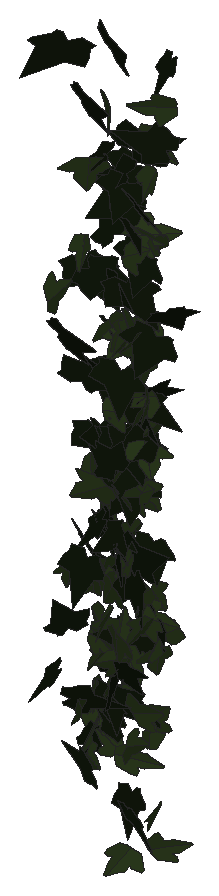
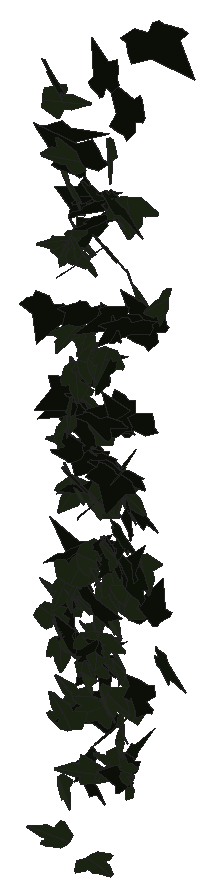
# SketchUp Ruby script. Lengths in inches.
U = 1.inch
M = Sketchup.active_model
def pt(a) = Geom::Point3d.new(a.map { |v| v * U })
def face(e, loops, mat)
  f = e.add_face(loops[0].map { |a| pt(a) })
  loops[1..].each { |l| e.add_face(l.map { |a| pt(a) }).erase! }
  f.material = f.back_material = mat if mat
  f
end
# faces: each face lists its corners as indices into pts; further lists are holes
def faces(e, pts, list, mat = nil) = list.each { |f| face(e, (f[0].is_a?(Array) ? f : [f]).map { |l| l.map { |i| pts[i] } }, mat) }
# xy, xz, yz: faces in a plane at the given z, y or x. An outline is a flat list of corners, or four numbers for a rectangle; further outlines are holes
def ring(l) = l.size == 4 ? [[l[0], l[1]], [l[2], l[1]], [l[2], l[3]], [l[0], l[3]]] : l.each_slice(2).to_a
def flat(e, list, mat, &to3) = list.each { |f| face(e, (f[0].is_a?(Array) ? f : [f]).map { |l| ring(l).map { |u, v| to3.(u, v) } }, mat) }
def xy(e, z, list, mat = nil) = flat(e, list, mat) { |x, y| [x, y, z] }
def xz(e, y, list, mat = nil) = flat(e, list, mat) { |x, z| [x, y, z] }
def yz(e, x, list, mat = nil) = flat(e, list, mat) { |y, z| [x, y, z] }
def lines(e, pts, list) = list.each { |a, b| e.add_line(pt(pts[a]), pt(pts[b])) }
# prism: a flat outline (further loops are holes) pulled along v
def prism(e, loops, v, mat = nil)
  f = face(e, loops, mat); d = Geom::Vector3d.new(v.map { |x| x * U })
  f.pushpull(f.normal.samedirection?(d) ? d.length : -d.length)
end
def box(e, o, s, mat = nil) = prism(e, [[o, [o[0] + s[0], o[1], o[2]], [o[0] + s[0], o[1] + s[1], o[2]], [o[0], o[1] + s[1], o[2]]]], [0, 0, s[2]], mat)
def at(x, y, z, deg = 0) = Geom::Transformation.translation(pt([x, y, z])) * Geom::Transformation.rotation(ORIGIN, Z_AXIS, deg.degrees)
def axes(o, x, y, z) = Geom::Transformation.new([*x, 0, *y, 0, *z, 0, *pt(o).to_a, 1])
def part(name) = M.definitions.add(name)
# library, detail: a bought-in or finely detailed component or shape, given as its bounding box
def library(name, o, s) = part(name).tap { |d| box(d.entities, o, s) }
def detail(e, o, s) = box(e.add_group.entities, o, s)
def put(e, d, t, mat = nil) = e.add_instance(d, t).tap { |i| i.material = mat if mat }
def group(e, t, mat = nil) = e.add_group.tap { |g| g.transformation = t; g.material = mat if mat }.entities
root = M.entities
M.materials.add("1026 AP 7946 SUNNY SIDE UP").color = [254, 231, 186]
M.materials.add("efeu1").color = [18, 25, 13]
M.materials.add("efeu2").color = [43, 57, 29]
c1 = part("ivyleaf_9")
p = [[1.54,2.16,1.25],[1.36,2.04,1.19],[-0.21,0.99,0.68],[-0.71,1.11,0.82],[-0.85,0.86,0.67],[-0.8,0.17,0.21],
  [-0.9,-0.01,0.1],[-0.67,-0.16,-0.02],[-0.08,-0.08,-0.05],[-0.03,-0.6,-0.4],[0.65,-0.88,-0.66],[0.83,-0.6,-0.49],
  [1.29,-0.42,-0.43],[1.8125,-0.07,-0.26],[1.21,0.44,0.15]]
faces(c1.entities,p,[[0,1,2,3,4,5,6,7,8,9,10,11,12,13,14]],"efeu1")
c2 = part("ivyleaf_10")
p = [[0,0.5,-0.03],[-0.0625,2.02,-0.43],[-0.19,2.01,-0.46],[-0.54,1.05,-0.29],[-0.52,0.625,-0.18],[-0.83,0.76,-0.28],
  [-1.16,0.64,-0.33],[-1.15,0.33,-0.24],[-0.77,-0.39,0.02],[-0.3,-0.51,0.16],[0.04,-0.48,0.23],[-0.02,2.01,-0.4375],
  [-0.06,2.01,-0.43],[0.04,-0.49,0.23],[0.67,-0.49,0.14],[1.38,0.36,-0.2],[1.375,0.51,-0.24],[0.81,0.65,-0.19],
  [0.62,0.59,-0.15],[0.6,1.09,-0.28],[0.5,1.23,-0.31]]
faces(c2.entities,p,[[0,1,2,3,4,5,6,7,8,9,10],[11,12,0,13,14,15,16,17,18,19,20]],"efeu2")
put(root,c1,axes([112.84,209.66,257.05],[-0.37781,-0.01782,-0.19523],[0.29911,-0.02649,-0.24619],[-0.00391,-0.3048,0.031]),"1026 AP 7946 SUNNY SIDE UP")
put(root,c1,axes([112.12,209.95,267.53],[0.03774,0.15785,-0.31881],[-0.06989,-0.30717,-0.16628],[-0.54303,0.0505,-0.00076]),"1026 AP 7946 SUNNY SIDE UP")
put(root,c1,axes([111.9375,210.06,261.28],[0.36942,-0.04727,-0.20032],[0.3095,0.00278,0.24465],[-0.05447,-0.30479,0.03148]),"1026 AP 7946 SUNNY SIDE UP")
put(root,c1,axes([111.83,210.03,254.21],[-0.27818,0.12757,-0.14576],[0.15899,-0.10192,-0.22437],[-0.25487,-0.20282,0.01912]),"1026 AP 7946 SUNNY SIDE UP")
put(root,c1,axes([112.01,210.17,255.13],[0.1892,0.0973,0.21691],[-0.29272,-0.09995,0.15701],[0.21625,-0.22043,0.02275]),"1026 AP 7946 SUNNY SIDE UP")
put(root,c1,axes([113.27,210.39,251.58],[0.18124,-0.20702,0.06487],[0.03095,-0.06236,-0.24411],[0.33938,0.11624,-0.01239]),"1026 AP 7946 SUNNY SIDE UP")
put(root,c2,axes([111.68,210.08,261.99],[0.03216,0.01268,-0.31587],[0.09557,0.30111,0.01876],[0.47309,-0.06169,0.01768]),"1026 AP 7946 SUNNY SIDE UP")
put(root,c2,axes([111.97,210.4,256.37],[-0.05548,-0.27655,0.01769],[0.00326,-0.01915,-0.28729],[0.43584,-0.03506,0.0044]),"1026 AP 7946 SUNNY SIDE UP")
put(root,c1,axes([112.28,210.46,252.09],[0.07837,-0.24976,0.04331],[0.0022,0.04456,0.26244],[-0.39862,-0.04886,0.00996]),"1026 AP 7946 SUNNY SIDE UP")
put(root,c2,axes([112.04,210.59,253.21],[-0.05761,-0.19311,-0.1727],[-0.02026,-0.16664,0.201],[-0.40046,0.03621,0.01467]),"1026 AP 7946 SUNNY SIDE UP")
put(root,c1,axes([112.03,210.59,266],[0.34896,-0.09762,-0.19804],[0.31181,-0.01386,0.24372],[-0.13105,-0.29292,0.05255]),"1026 AP 7946 SUNNY SIDE UP")
put(root,c2,axes([112.98,210.43,255.11],[-0.33435,0.15157,0.06874],[-0.10884,0.01577,-0.26753],[-0.23596,-0.22205,0.026]),"1026 AP 7946 SUNNY SIDE UP")
put(root,c1,axes([112.84,210.66,260.55],[-0.12699,-0.28062,-0.00455],[0.019,-0.00055,-0.30059],[0.44087,-0.08081,0.01165]),"1026 AP 7946 SUNNY SIDE UP")
put(root,c1,axes([111.92,210.43,253.47],[0.22646,0.03739,0.22439],[0.3424,0.01889,-0.15171],[-0.05738,0.26026,-0.01967]),"1026 AP 7946 SUNNY SIDE UP")
put(root,c2,axes([113.29,210.37,253],[-0.02217,-0.10445,-0.24966],[0.10453,0.23284,-0.10627],[0.40067,-0.06652,0.01391]),"1026 AP 7946 SUNNY SIDE UP")
put(root,c1,axes([112.625,210.7,253.7],[0.04338,0.11867,0.27502],[-0.12079,-0.25506,0.12381],[0.4422,-0.08131,0.00684]),"1026 AP 7946 SUNNY SIDE UP")
put(root,c2,axes([112.4,210.63,257.99],[-0.26989,-0.0335,0.21812],[-0.3125,-0.07742,-0.17889],[0.1271,-0.26149,0.02333]),"1026 AP 7946 SUNNY SIDE UP")
put(root,c2,axes([113.35,210.74,255.42],[-0.00839,-0.21307,0.16183],[-0.00922,-0.1582,-0.22049],[0.41727,-0.00778,-0.00162]),"1026 AP 7946 SUNNY SIDE UP")
put(root,c2,axes([112.68,210.85,254.4],[-0.00264,0.07244,0.29267],[0.05489,-0.28161,0.07265],[0.45709,0.03424,-0.00703]),"1026 AP 7946 SUNNY SIDE UP")
put(root,c2,axes([112.46,210.76,255.29],[0.14967,-0.25162,0.0702],[0.02316,-0.06876,-0.27734],[0.40983,0.09578,-0.00997]),"1026 AP 7946 SUNNY SIDE UP")
put(root,c2,axes([112.97,210.76,263],[0.1487,-0.16465,-0.18246],[0.22404,-0.11452,0.18838],[-0.30591,-0.16391,0.04927]),"1026 AP 7946 SUNNY SIDE UP")
put(root,c2,axes([113.52,210.57,260.18],[0.12239,-0.21871,-0.18692],[-0.03173,0.18212,-0.23563],[0.44446,0.07323,0.03465]),"1026 AP 7946 SUNNY SIDE UP")
put(root,c1,axes([112.28,210.79,257.17],[-0.29222,0.11367,-0.13312],[0.1565,-0.08531,-0.22417],[-0.2217,-0.21006,0.01721]),"1026 AP 7946 SUNNY SIDE UP")
put(root,c1,axes([112.95,210.84,251.65],[-0.27007,-0.00097,-0.21958],[0.33276,-0.03334,-0.17573],[-0.03987,-0.27169,0.02073]),"1026 AP 7946 SUNNY SIDE UP")
put(root,c1,axes([112.73,210.61,258.52],[-0.06344,0.11746,0.2405],[-0.21429,0.19132,-0.12267],[-0.34953,-0.13861,0.03155]),"1026 AP 7946 SUNNY SIDE UP")
put(root,c1,axes([112.97,210.89,264.03],[0.18064,-0.158,0.17429],[0.14243,-0.14422,-0.20189],[0.33609,0.14603,-0.00812]),"1026 AP 7946 SUNNY SIDE UP")
put(root,c1,axes([112.67,210.71,254.3],[0.37853,0.07605,-0.02641],[-0.02774,-0.03032,-0.25913],[-0.12333,0.24023,-0.02278]),"1026 AP 7946 SUNNY SIDE UP")
put(root,c2,axes([112.98,211.01,261.03],[-0.0252,-0.02202,-0.27195],[-0.0797,-0.2592,0.02394],[-0.40863,0.05191,0.0121]),"1026 AP 7946 SUNNY SIDE UP")
put(root,c1,axes([112.73,210.99,264.29],[-0.18941,-0.22515,0.03642],[-0.00694,-0.03912,-0.26287],[0.35861,-0.11968,0.01415]),"1026 AP 7946 SUNNY SIDE UP")
put(root,c1,axes([112.92,210.98,256.07],[-0.15698,-0.00274,-0.28617],[0.42715,-0.06264,-0.10031],[-0.09127,-0.28845,0.02274]),"1026 AP 7946 SUNNY SIDE UP")
put(root,c2,axes([112.66,210.86,257.61],[-0.35606,0.06259,-0.09732],[-0.14008,0.03343,0.24209],[0.11089,0.24321,-0.00669]),"1026 AP 7946 SUNNY SIDE UP")
put(root,c1,axes([112.01,210.91,256.34],[0.15561,-0.195,0.1244],[-0.06835,0.11441,0.22564],[-0.35504,-0.10749,0.01108]),"1026 AP 7946 SUNNY SIDE UP")
put(root,c1,axes([112.55,211.03,256.19],[-0.02223,0.02678,0.2683],[-0.06207,-0.2579,0.02362],[0.40672,-0.03789,0.01827]),"1026 AP 7946 SUNNY SIDE UP")
put(root,c2,axes([111.67,211,262.73],[0.27923,-0.12257,0.13379],[0.1415,-0.0979,-0.22134],[0.24346,0.19748,-0.02481]),"1026 AP 7946 SUNNY SIDE UP")
put(root,c1,axes([113.34,211.05,261.26],[-0.28684,-0.20836,0.00178],[0.01744,-0.01357,-0.28482],[0.3272,-0.18194,0.01674]),"1026 AP 7946 SUNNY SIDE UP")
put(root,c2,axes([112.15,211.07,255.88],[-0.10938,-0.1675,0.2339],[-0.0872,-0.22216,-0.18687],[0.43622,-0.08641,0.02129]),"1026 AP 7946 SUNNY SIDE UP")
put(root,c1,axes([112.62,211.11,263.54],[0.05658,-0.24355,0.19518],[0.09902,-0.18235,-0.25303],[0.47634,0.06684,0.02941]),"1026 AP 7946 SUNNY SIDE UP")
put(root,c2,axes([112.52,210.83,255.8],[-0.27627,0.11066,0.14898],[-0.21598,0.05008,-0.21202],[-0.18679,-0.22157,0.0248]),"1026 AP 7946 SUNNY SIDE UP")
put(root,c2,axes([111.97,210.89,255.65],[-0.35034,0.09214,-0.06741],[-0.08307,0.04426,0.24779],[0.15763,0.22811,-0.01924]),"1026 AP 7946 SUNNY SIDE UP")
put(root,c1,axes([112.32,211.08,253.41],[0.01865,-0.24583,0.08658],[0.0049,-0.08539,-0.25405],[0.4092,0.01222,-0.0009]),"1026 AP 7946 SUNNY SIDE UP")
put(root,c1,axes([113.57,211.01,265.32],[-0.14562,0.02578,0.25128],[-0.38371,-0.03438,-0.09196],[0.03651,-0.25849,0.03573]),"1026 AP 7946 SUNNY SIDE UP")
put(root,c2,axes([112.21,210.97,256.2],[-0.10157,-0.27266,0.017],[0.00408,-0.01916,-0.2887],[0.42966,-0.06427,0.00676]),"1026 AP 7946 SUNNY SIDE UP")
put(root,c1,axes([112.96,211.17,262.8],[-0.09542,-0.27001,0.14839],[-0.01855,-0.14623,-0.28534],[0.48198,-0.05908,0.01839]),"1026 AP 7946 SUNNY SIDE UP")
put(root,c2,axes([113.16,211.02,255.37],[0.06627,-0.09094,-0.28766],[0.39227,-0.13679,0.08404],[-0.24215,-0.24647,0.05741]),"1026 AP 7946 SUNNY SIDE UP")
put(root,c1,axes([112.27,211.13,266.92],[-0.04107,-0.05187,0.32342],[0.14049,-0.30382,-0.04579],[0.48068,0.08437,0.04102]),"1026 AP 7946 SUNNY SIDE UP")
put(root,c2,axes([112.95,211.07,257.82],[0.1335,-0.17886,-0.2004],[0.18869,-0.15476,0.2007],[-0.36889,-0.14389,0.03013]),"1026 AP 7946 SUNNY SIDE UP")
put(root,c1,axes([112.51,211.15,256.85],[0.03964,-0.0827,-0.23533],[0.10634,-0.2177,0.08779],[-0.36618,-0.07218,0.00002]),"1026 AP 7946 SUNNY SIDE UP")
put(root,c2,axes([113.39,210.875,252.9],[0.27964,-0.09049,0.1386],[-0.16708,0.08679,0.20456],[-0.19346,-0.20576,0.02368]),"1026 AP 7946 SUNNY SIDE UP")
put(root,c2,axes([112.99,210.99,253.29],[-0.23492,0.01676,0.22293],[0.34026,-0.00724,0.15451],[0.02435,0.26278,-0.00841]),"1026 AP 7946 SUNNY SIDE UP")
put(root,c2,axes([111.73,211.1,252],[-0.03774,-0.00188,-0.25255],[0.20852,-0.20726,-0.01295],[-0.3242,-0.13309,0.02107]),"1026 AP 7946 SUNNY SIDE UP")
put(root,c2,axes([113.41,211.01,251.41],[0.06828,-0.231,0.01425],[-0.00237,-0.01569,-0.2422],[0.364,0.04323,-0.00425]),"1026 AP 7946 SUNNY SIDE UP")
put(root,c1,axes([111.57,210.9375,256.24],[0.05252,0.25673,0.11278],[-0.02706,-0.10668,0.26606],[0.43711,-0.03745,0.00292]),"1026 AP 7946 SUNNY SIDE UP")
put(root,c2,axes([113.03,211.18,255.59],[-0.03088,0.04404,0.28941],[0.20147,-0.24974,0.04814],[0.39873,0.1296,-0.00191]),"1026 AP 7946 SUNNY SIDE UP")
put(root,c1,axes([112.59,211.23,263.87],[-0.27402,-0.1595,0.21147],[-0.16452,-0.18436,-0.23911],[0.37542,-0.19721,0.04957]),"1026 AP 7946 SUNNY SIDE UP")
put(root,c1,axes([112.82,211.07,256.41],[-0.01565,0.03491,0.30244],[0.26687,-0.23959,0.0339],[0.38025,0.16959,-0.01134]),"1026 AP 7946 SUNNY SIDE UP")
put(root,c2,axes([112.33,211.07,253.71],[0.14097,-0.24887,0.04596],[0.01492,-0.04548,-0.2727],[0.39768,0.08993,-0.00606]),"1026 AP 7946 SUNNY SIDE UP")
put(root,c2,axes([111.82,211.01,264.42],[-0.29463,-0.23869,-0.00195],[0.01934,-0.00897,-0.31227],[0.37482,-0.18716,0.01457]),"1026 AP 7946 SUNNY SIDE UP")
put(root,c1,axes([112.77,211.15,258.13],[-0.19524,-0.27925,-0.03537],[0.03825,0.02499,-0.31445],[0.44045,-0.12596,0.01163]),"1026 AP 7946 SUNNY SIDE UP")
put(root,c2,axes([113.56,211.125,266.15],[0.00784,0.02496,-0.26823],[-0.3641,-0.12098,-0.01722],[-0.19173,0.23077,0.02173]),"1026 AP 7946 SUNNY SIDE UP")
put(root,c2,axes([113.13,211.02,258.89],[0.3314,0.13721,0.04512],[0.07258,0.00773,-0.25834],[-0.21413,0.21496,-0.01774]),"1026 AP 7946 SUNNY SIDE UP")
put(root,c2,axes([112.47,211.19,258.01],[0.11625,-0.22378,0.18462],[0.08425,-0.17236,-0.24378],[0.44413,0.09127,-0.00208]),"1026 AP 7946 SUNNY SIDE UP")
put(root,c1,axes([112.52,211.28,257.79],[-0.09589,-0.21996,0.21179],[-0.07847,-0.20077,-0.23628],[0.46823,-0.07869,0.00378]),"1026 AP 7946 SUNNY SIDE UP")
put(root,c2,axes([113.15,211.04,259.98],[0.22212,-0.02104,-0.2187],[-0.3311,0.02617,-0.14695],[0.0526,0.25355,-0.00147]),"1026 AP 7946 SUNNY SIDE UP")
put(root,c2,axes([112.7,211.05,256.41],[0.2345,-0.20168,-0.04669],[-0.06035,0.02647,-0.25779],[0.31899,0.15327,-0.01445]),"1026 AP 7946 SUNNY SIDE UP")
put(root,c1,axes([113.12,211.11,259.04],[-0.44106,0.05807,-0.046],[0.05993,-0.03671,-0.29391],[-0.09874,-0.2817,0.02708]),"1026 AP 7946 SUNNY SIDE UP")
put(root,c2,axes([112.61,210.98,254.76],[0.33913,-0.1294,0.07505],[-0.07865,0.05903,0.25828],[-0.22046,-0.22011,0.02331]),"1026 AP 7946 SUNNY SIDE UP")
put(root,c1,axes([112.49,210.89,263.26],[-0.2956,0.06199,-0.16776],[-0.22714,0.07943,0.20298],[0.15414,0.23594,-0.02262]),"1026 AP 7946 SUNNY SIDE UP")
put(root,c2,axes([111.71,211.21,258.1],[0.21782,-0.10008,0.22974],[0.24337,-0.16332,-0.17506],[0.29853,0.20616,-0.02492]),"1026 AP 7946 SUNNY SIDE UP")
put(root,c1,axes([112.39,211.14,252.76],[-0.06125,-0.24874,0.07028],[0.01073,0.06941,0.25975],[-0.40601,0.03936,-0.00374]),"1026 AP 7946 SUNNY SIDE UP")
put(root,c2,axes([113.14,211.16,264.54],[0.30456,-0.22569,0.04364],[0.01776,-0.04765,-0.30581],[0.36101,0.19274,-0.02177]),"1026 AP 7946 SUNNY SIDE UP")
put(root,c2,axes([112.58,211.17,250.13],[0.22664,0.14036,-0.16224],[-0.16696,-0.11766,-0.20778],[-0.28771,0.17884,-0.00723]),"1026 AP 7946 SUNNY SIDE UP")
put(root,c1,axes([111.99,211.29,258.54],[0.14663,-0.22853,-0.12501],[0.11114,-0.10016,0.2524],[-0.3904,-0.11435,0.0249]),"1026 AP 7946 SUNNY SIDE UP")
put(root,c2,axes([112.3125,211.1,259.36],[0.07051,-0.05906,-0.24778],[0.37777,-0.04761,0.05799],[-0.09242,-0.23965,0.048]),"1026 AP 7946 SUNNY SIDE UP")
put(root,c2,axes([111.77,211.06,252.24],[0.16143,-0.23906,0.06526],[-0.02497,0.06354,0.26819],[-0.38862,-0.10338,0.00988]),"1026 AP 7946 SUNNY SIDE UP")
put(root,c2,axes([111.76,211.22,253.2],[0.03157,0.01393,0.25321],[0.31201,-0.14674,-0.00899],[0.2289,0.19809,-0.02267]),"1026 AP 7946 SUNNY SIDE UP")
put(root,c1,axes([113.38,211.01,255.43],[0.1385,-0.00669,-0.25103],[-0.38215,0.01712,-0.0909],[0.02889,0.2585,0.00104]),"1026 AP 7946 SUNNY SIDE UP")
put(root,c2,axes([112.6,211.29,254.18],[0.11275,-0.14177,0.22476],[0.14612,-0.19832,-0.16479],[0.38328,0.11731,-0.0033]),"1026 AP 7946 SUNNY SIDE UP")
put(root,c2,axes([112.58,211.14,254.35],[0.34975,0.03537,0.1412],[0.21784,-0.0039,-0.23095],[-0.04411,0.26113,-0.02102]),"1026 AP 7946 SUNNY SIDE UP")
put(root,c1,axes([112.63,211.05,264.48],[-0.23768,0.20229,0.05341],[-0.07807,0.0259,-0.25884],[-0.31848,-0.15732,0.02359]),"1026 AP 7946 SUNNY SIDE UP")
put(root,c2,axes([113.02,211.04,257.97],[-0.219,-0.20117,-0.15201],[0.16277,0.10573,-0.25048],[0.35576,-0.17221,0.02102]),"1026 AP 7946 SUNNY SIDE UP")
put(root,c1,axes([111.99,211.25,256.79],[0.17543,-0.21172,0.12165],[0.06829,-0.11177,-0.24688],[0.37596,0.1191,-0.01192]),"1026 AP 7946 SUNNY SIDE UP")
put(root,c2,axes([112.97,211.13,260.51],[-0.1553,-0.27376,-0.02504],[0.0255,0.01832,-0.29956],[0.43119,-0.09968,0.0087]),"1026 AP 7946 SUNNY SIDE UP")
put(root,c2,axes([111.79,211.22,254.43],[0.05098,0.00828,0.2655],[0.38382,-0.08454,-0.02934],[0.13042,0.24556,-0.01744]),"1026 AP 7946 SUNNY SIDE UP")
put(root,c1,axes([112.57,211.18,258.875],[-0.21877,-0.15663,-0.20244],[0.2261,0.13335,-0.21457],[0.32272,-0.1996,0.0131]),"1026 AP 7946 SUNNY SIDE UP")
put(root,c2,axes([113.12,211.24,263.04],[-0.25773,-0.13628,-0.14152],[-0.149,-0.09929,0.21859],[-0.2643,0.18886,0.01478]),"1026 AP 7946 SUNNY SIDE UP")
put(root,c1,axes([111.9,211.2,258.78],[-0.19978,-0.1483,-0.21529],[0.28549,0.11121,-0.19516],[0.28282,-0.21702,0.04492]),"1026 AP 7946 SUNNY SIDE UP")
put(root,c1,axes([112.625,211.3125,254.59],[-0.13649,-0.03333,0.23754],[-0.28054,-0.14904,-0.09219],[0.23604,-0.19641,0.0278]),"1026 AP 7946 SUNNY SIDE UP")
put(root,c1,axes([111.94,211.28,256.94],[-0.05938,-0.04917,-0.26042],[0.39716,-0.0555,-0.02811],[-0.07673,-0.24922,0.05605]),"1026 AP 7946 SUNNY SIDE UP")
put(root,c2,axes([112.55,211.21,261.37],[-0.19877,0.17616,-0.13537],[0.09232,-0.1202,-0.2232],[-0.33398,-0.13807,0.01887]),"1026 AP 7946 SUNNY SIDE UP")
put(root,c2,axes([112.46,211.15,254.9],[-0.3657,-0.15825,-0.0097],[0.03105,-0.01394,-0.28894],[0.24725,-0.23231,0.02194]),"1026 AP 7946 SUNNY SIDE UP")
put(root,c1,axes([112.79,211.14,265.02],[-0.04459,0.00137,0.31293],[0.44254,-0.11464,0.02693],[0.17967,0.28271,0.01133]),"1026 AP 7946 SUNNY SIDE UP")
put(root,c1,axes([112.95,211.07,259.8125],[0.00444,-0.07237,-0.25204],[0.13806,0.22956,-0.06769],[0.376,-0.08344,0.02783]),"1026 AP 7946 SUNNY SIDE UP")
put(root,c2,axes([113.27,211.11,254.61],[0.23155,-0.20943,0.07667],[-0.02919,0.07879,0.26252],[-0.34889,-0.14558,0.02892]),"1026 AP 7946 SUNNY SIDE UP")
put(root,c2,axes([111.87,211.17,258.17],[-0.01952,0.2455,-0.05051],[-0.00122,-0.05052,-0.25351],[-0.39408,-0.01201,0.00328]),"1026 AP 7946 SUNNY SIDE UP")
put(root,c1,axes([111.72,211.23,259.99],[0.3155,-0.14068,0.15187],[0.16583,-0.10663,-0.25197],[0.27522,0.22552,-0.02228]),"1026 AP 7946 SUNNY SIDE UP")
put(root,c1,axes([112.41,211.08,253.38],[0.00837,-0.04478,-0.27289],[0.20959,0.23018,-0.03602],[0.36631,-0.13068,0.02685]),"1026 AP 7946 SUNNY SIDE UP")
put(root,c1,axes([111.6,211.13,259.75],[-0.18937,-0.00565,0.24602],[0.36874,-0.05391,0.12019],[0.07178,0.262,0.03163]),"1026 AP 7946 SUNNY SIDE UP")
put(root,c2,axes([112.91,211.29,256.17],[-0.26029,-0.18983,-0.13709],[-0.16221,-0.08465,0.25819],[-0.32536,0.19406,-0.01905]),"1026 AP 7946 SUNNY SIDE UP")
put(root,c2,axes([113.58,211.25,255.15],[-0.18572,-0.02645,0.21552],[-0.28439,-0.1109,-0.1202],[0.17092,-0.21326,0.03418]),"1026 AP 7946 SUNNY SIDE UP")
put(root,c2,axes([112.42,211.18,253.46],[-0.28482,-0.02547,-0.17583],[0.27031,-0.00767,-0.18698],[0.02084,-0.24866,0.02231]),"1026 AP 7946 SUNNY SIDE UP")
put(root,c2,axes([113.22,211.125,255.86],[-0.09538,-0.2302,-0.14715],[0.12036,0.12448,-0.24164],[0.4075,-0.09065,0.03693]),"1026 AP 7946 SUNNY SIDE UP")
put(root,c1,axes([111.98,211.3,261.9375],[0.06914,-0.06862,-0.24408],[0.38727,0.01207,0.04363],[-0.00029,-0.24029,0.07038]),"1026 AP 7946 SUNNY SIDE UP")
put(root,c1,axes([111.74,211.05,257.63],[0.04138,-0.02262,0.25358],[0.08166,0.24265,0.01866],[-0.38021,0.04965,0.03161]),"1026 AP 7946 SUNNY SIDE UP")
put(root,c2,axes([113.28,211.22,254.56],[-0.14781,-0.23215,-0.02346],[0.02798,0.01592,-0.25771],[0.36552,-0.0951,0.01024]),"1026 AP 7946 SUNNY SIDE UP")
put(root,c2,axes([112.51,211.43,260.99],[0.01753,-0.15011,0.26796],[0.0829,-0.25613,-0.1556],[0.46607,0.0512,0.0176]),"1026 AP 7946 SUNNY SIDE UP")
put(root,c1,axes([112.55,211.33,259.55],[0.03895,-0.02593,-0.30476],[0.4655,-0.01922,0.02717],[-0.03363,-0.29609,0.02317]),"1026 AP 7946 SUNNY SIDE UP")
put(root,c2,axes([112.46,211.29,260.91],[0.30727,0.11915,-0.11173],[-0.129,-0.07437,-0.23543],[-0.21888,0.21111,-0.0181]),"1026 AP 7946 SUNNY SIDE UP")
put(root,c1,axes([112.03,211.21,264.59],[-0.24576,0.1988,-0.028],[0.00571,-0.03307,-0.26009],[-0.3157,-0.15536,0.0171]),"1026 AP 7946 SUNNY SIDE UP")
put(root,c2,axes([113.04,211.11,259.71],[-0.00479,-0.20851,-0.20891],[0.01524,0.20143,-0.21359],[0.45579,-0.00893,0.00495]),"1026 AP 7946 SUNNY SIDE UP")
put(root,c1,axes([112.8,211.19,254.61],[-0.24063,0.0658,0.21109],[0.29507,-0.08135,0.17113],[0.16452,0.24214,0.00181]),"1026 AP 7946 SUNNY SIDE UP")
put(root,c1,axes([112.5625,211.23,262.04],[-0.06264,-0.19881,-0.22015],[0.10636,0.20235,-0.20685],[0.44512,-0.07633,0.01845]),"1026 AP 7946 SUNNY SIDE UP")
put(root,c2,axes([112.34,211.41,261.04],[0.04267,-0.1782,0.19161],[0.08486,-0.17997,-0.1858],[0.39721,0.0576,0.01911]),"1026 AP 7946 SUNNY SIDE UP")
put(root,c2,axes([112.19,211.18,261.13],[-0.09065,-0.24731,-0.14591],[0.11065,0.12622,-0.25838],[0.43312,-0.08401,0.03547]),"1026 AP 7946 SUNNY SIDE UP")
put(root,c1,axes([112.83,211.16,258.7],[-0.3347,0.00378,0.1848],[0.28121,0.02639,0.21823],[-0.02222,0.27709,-0.02167]),"1026 AP 7946 SUNNY SIDE UP")
put(root,c1,axes([111.74,211.08,252.2],[0.00331,0.03687,0.26194],[0.27533,0.18558,-0.02816],[-0.29518,0.17351,-0.02332]),"1026 AP 7946 SUNNY SIDE UP")
put(root,c2,axes([112.15,211.34,252.17],[-0.00692,0.20322,0.1357],[-0.01047,-0.13064,0.20848],[0.37968,0.0001,0.00822]),"1026 AP 7946 SUNNY SIDE UP")
put(root,c2,axes([112.99,211.08,263.3125],[0.10786,-0.07001,-0.30579],[0.33505,0.22816,-0.00338],[0.34223,-0.2013,0.09969]),"1026 AP 7946 SUNNY SIDE UP")
put(root,c2,axes([112.54,211.45,256.8125],[0.03812,-0.15596,0.22328],[0.03777,-0.21637,-0.16376],[0.41929,0.03367,-0.00555]),"1026 AP 7946 SUNNY SIDE UP")
put(root,c2,axes([113.09,211.46,259.24],[-0.00333,0.00383,0.26467],[0.12958,-0.24332,0.00302],[0.38264,0.08243,0.00128]),"1026 AP 7946 SUNNY SIDE UP")
put(root,c1,axes([113.03,211.4,256.69],[-0.06162,-0.2497,-0.0068],[0.00853,0.00439,-0.26032],[0.39262,-0.03929,0.00459]),"1026 AP 7946 SUNNY SIDE UP")
put(root,c1,axes([111.79,211.14,262.12],[0.11426,-0.06583,-0.28922],[0.03712,0.28955,-0.06204],[0.45133,-0.00715,0.07832]),"1026 AP 7946 SUNNY SIDE UP")
put(root,c2,axes([112.14,211.16,265.61],[0.20298,-0.18707,-0.22568],[-0.06091,0.22549,-0.22164],[0.44757,0.11553,0.07219]),"1026 AP 7946 SUNNY SIDE UP")
put(root,c1,axes([111.53,211.29,262.11],[-0.00092,-0.2282,-0.20852],[0.09275,0.19721,-0.22955],[0.4692,-0.03943,0.04497]),"1026 AP 7946 SUNNY SIDE UP")
put(root,c2,axes([111.88,211.44,257.06],[-0.07587,0.00698,-0.23906],[0.20075,-0.1972,-0.03461],[-0.30496,-0.13155,0.03669]),"1026 AP 7946 SUNNY SIDE UP")
put(root,c2,axes([113,211.33,253.03],[-0.34786,-0.01497,0.14592],[0.22038,0.0246,0.2282],[-0.04064,0.26158,-0.01156]),"1026 AP 7946 SUNNY SIDE UP")
put(root,c1,axes([113.13,211.12,259.95],[0.15381,0.14281,0.19838],[0.19458,0.14703,-0.17698],[-0.32167,0.15723,-0.0122]),"1026 AP 7946 SUNNY SIDE UP")
put(root,c1,axes([113.39,211.43,266.93],[-0.26923,0.05718,-0.1936],[0.25833,-0.09574,-0.18446],[-0.17019,-0.23577,0.02626]),"1026 AP 7946 SUNNY SIDE UP")
put(root,c2,axes([112.88,211.34,265.19],[0.14931,0.03455,0.26791],[0.4097,0.01799,-0.10044],[-0.04538,0.27608,-0.02533]),"1026 AP 7946 SUNNY SIDE UP")
put(root,c2,axes([112.98,211.25,261.42],[0.09872,0.22937,0.09862],[0.05276,0.08866,-0.24431],[-0.38644,0.0707,-0.00816]),"1026 AP 7946 SUNNY SIDE UP")
put(root,c1,axes([112.52,211.21,255.64],[-0.04955,0.06909,0.27169],[-0.2293,0.21957,-0.07604],[-0.36149,-0.14875,0.01099]),"1026 AP 7946 SUNNY SIDE UP")
put(root,c2,axes([111.625,211.52,253.16],[0.07353,-0.10491,0.24022],[0.20478,-0.19493,-0.1181],[0.34699,0.13727,0.01879]),"1026 AP 7946 SUNNY SIDE UP")
put(root,c1,axes([112.125,211.45,259.9],[-0.31759,-0.15419,-0.11496],[0.15965,0.04883,-0.26061],[0.25219,-0.2251,0.02021]),"1026 AP 7946 SUNNY SIDE UP")
put(root,c1,axes([112.46,211.55,264.36],[-0.19039,-0.20814,0.12175],[-0.07495,-0.11017,-0.24837],[0.36976,-0.1295,0.01235]),"1026 AP 7946 SUNNY SIDE UP")
put(root,c2,axes([113.15,211.31,263.02],[-0.16367,0.23077,-0.04307],[-0.03024,0.03862,0.26102],[0.36789,0.10584,0.0023]),"1026 AP 7946 SUNNY SIDE UP")
put(root,c1,axes([111.98,211.43,260.88],[0.24505,-0.19861,0.05492],[0.02828,-0.05488,-0.25964],[0.32257,0.15569,-0.01895]),"1026 AP 7946 SUNNY SIDE UP")
put(root,c2,axes([111.62,211.49,254.71],[-0.07359,0.04129,-0.23088],[0.16383,-0.19986,-0.06146],[-0.31908,-0.11214,0.02169]),"1026 AP 7946 SUNNY SIDE UP")
put(root,c1,axes([113.49,211.22,261.76],[0.21237,0.22001,0.01049],[0.02539,0.00055,-0.26559],[-0.3453,0.13536,-0.01308]),"1026 AP 7946 SUNNY SIDE UP")
put(root,c2,axes([112.52,211.47,263.28],[0.30652,-0.08218,0.20204],[0.2643,-0.10444,-0.2173],[0.2059,0.2564,-0.02185]),"1026 AP 7946 SUNNY SIDE UP")
put(root,c2,axes([111.79,211.49,254.02],[0.01029,-0.1848,0.13991],[0.00185,-0.13689,-0.19128],[0.36159,0.00596,-0.003]),"1026 AP 7946 SUNNY SIDE UP")
put(root,c2,axes([112.47,211.26,252.08],[0.00602,0.02139,0.25634],[0.29708,0.16232,-0.01642],[-0.25653,0.18848,-0.01301]),"1026 AP 7946 SUNNY SIDE UP")
put(root,c1,axes([111.9375,211.24,258.65],[0.17907,0.22343,-0.00136],[0.01315,-0.00716,-0.25816],[-0.35111,0.11369,-0.01036]),"1026 AP 7946 SUNNY SIDE UP")
put(root,c1,axes([112.9,211.39,258.4],[-0.38796,0.15385,-0.00752],[-0.00905,-0.02463,-0.29867],[-0.24208,-0.24564,0.02322]),"1026 AP 7946 SUNNY SIDE UP")
put(root,c2,axes([113.24,211.27,250.41],[-0.1168,-0.06474,0.22197],[0.21369,0.1684,0.10121],[-0.28262,0.15408,-0.01521]),"1026 AP 7946 SUNNY SIDE UP")
put(root,c2,axes([111.79,211.33,252.52],[0.38319,0.03651,0.00958],[-0.01959,0.02209,0.25281],[0.05582,-0.24287,0.02297]),"1026 AP 7946 SUNNY SIDE UP")
